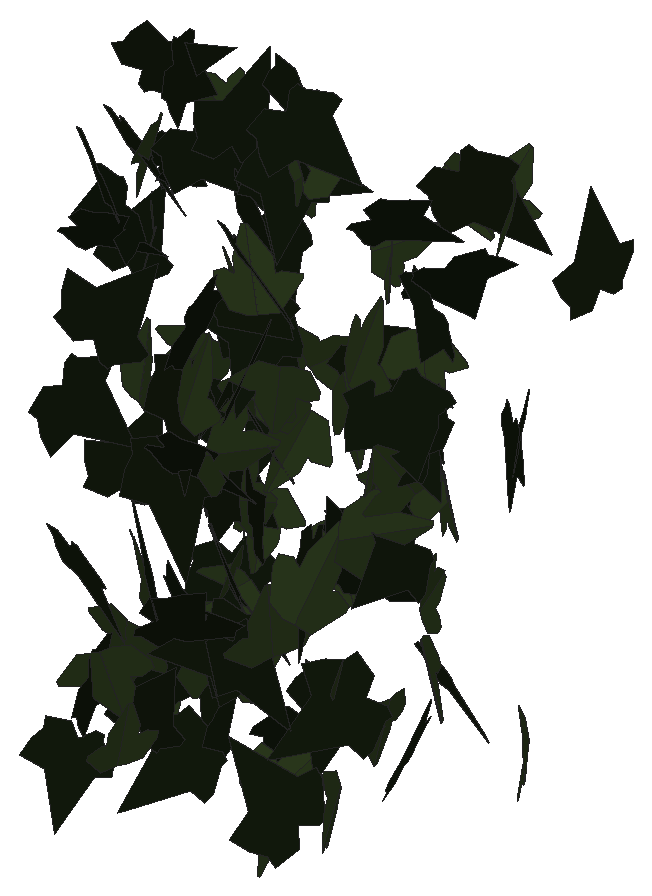
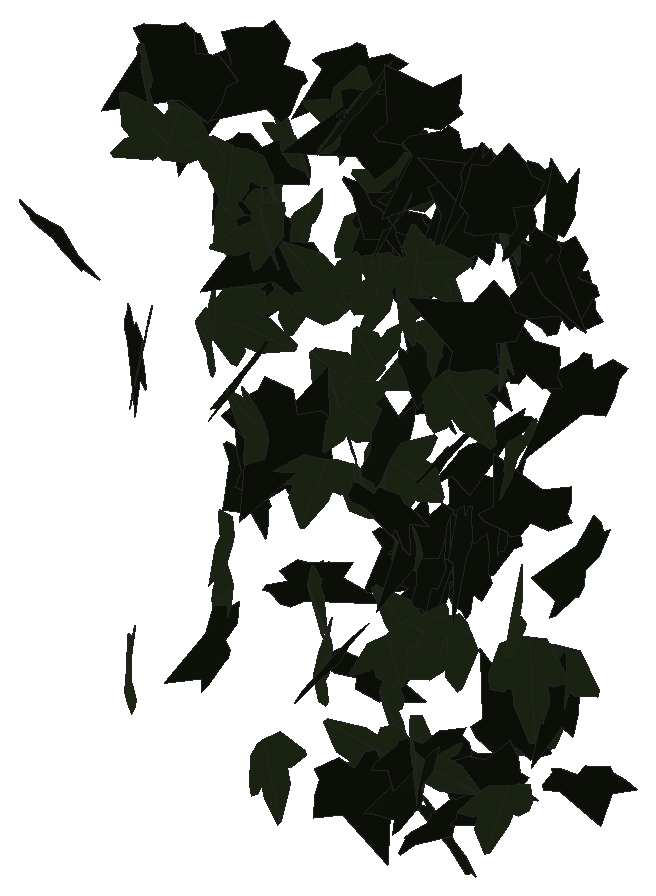
# SketchUp Ruby script. Lengths in inches.
U = 1.inch
M = Sketchup.active_model
def pt(a) = Geom::Point3d.new(a.map { |v| v * U })
def face(e, loops, mat)
  f = e.add_face(loops[0].map { |a| pt(a) })
  loops[1..].each { |l| e.add_face(l.map { |a| pt(a) }).erase! }
  f.material = f.back_material = mat if mat
  f
end
# faces: each face lists its corners as indices into pts; further lists are holes
def faces(e, pts, list, mat = nil) = list.each { |f| face(e, (f[0].is_a?(Array) ? f : [f]).map { |l| l.map { |i| pts[i] } }, mat) }
# xy, xz, yz: faces in a plane at the given z, y or x. An outline is a flat list of corners, or four numbers for a rectangle; further outlines are holes
def ring(l) = l.size == 4 ? [[l[0], l[1]], [l[2], l[1]], [l[2], l[3]], [l[0], l[3]]] : l.each_slice(2).to_a
def flat(e, list, mat, &to3) = list.each { |f| face(e, (f[0].is_a?(Array) ? f : [f]).map { |l| ring(l).map { |u, v| to3.(u, v) } }, mat) }
def xy(e, z, list, mat = nil) = flat(e, list, mat) { |x, y| [x, y, z] }
def xz(e, y, list, mat = nil) = flat(e, list, mat) { |x, z| [x, y, z] }
def yz(e, x, list, mat = nil) = flat(e, list, mat) { |y, z| [x, y, z] }
def lines(e, pts, list) = list.each { |a, b| e.add_line(pt(pts[a]), pt(pts[b])) }
# prism: a flat outline (further loops are holes) pulled along v
def prism(e, loops, v, mat = nil)
  f = face(e, loops, mat); d = Geom::Vector3d.new(v.map { |x| x * U })
  f.pushpull(f.normal.samedirection?(d) ? d.length : -d.length)
end
def box(e, o, s, mat = nil) = prism(e, [[o, [o[0] + s[0], o[1], o[2]], [o[0] + s[0], o[1] + s[1], o[2]], [o[0], o[1] + s[1], o[2]]]], [0, 0, s[2]], mat)
def at(x, y, z, deg = 0) = Geom::Transformation.translation(pt([x, y, z])) * Geom::Transformation.rotation(ORIGIN, Z_AXIS, deg.degrees)
def axes(o, x, y, z) = Geom::Transformation.new([*x, 0, *y, 0, *z, 0, *pt(o).to_a, 1])
def part(name) = M.definitions.add(name)
# library, detail: a bought-in or finely detailed component or shape, given as its bounding box
def library(name, o, s) = part(name).tap { |d| box(d.entities, o, s) }
def detail(e, o, s) = box(e.add_group.entities, o, s)
def put(e, d, t, mat = nil) = e.add_instance(d, t).tap { |i| i.material = mat if mat }
def group(e, t, mat = nil) = e.add_group.tap { |g| g.transformation = t; g.material = mat if mat }.entities
root = M.entities
M.materials.add("efeu1").color = [18, 25, 13]
M.materials.add("efeu2").color = [43, 57, 29]
c1 = part("ivyleaf_9")
p = [[1.54,2.16,1.25],[1.36,2.04,1.19],[-0.21,0.99,0.68],[-0.71,1.11,0.82],[-0.85,0.86,0.67],[-0.8,0.17,0.21],
  [-0.9,-0.01,0.1],[-0.67,-0.16,-0.02],[-0.08,-0.08,-0.05],[-0.03,-0.6,-0.4],[0.65,-0.88,-0.66],[0.83,-0.6,-0.49],
  [1.29,-0.42,-0.43],[1.8125,-0.07,-0.26],[1.21,0.44,0.15]]
faces(c1.entities,p,[[0,1,2,3,4,5,6,7,8,9,10,11,12,13,14]],"efeu1")
c2 = part("ivyleaf_10")
p = [[0,0.5,-0.03],[-0.0625,2.02,-0.43],[-0.19,2.01,-0.46],[-0.54,1.05,-0.29],[-0.52,0.625,-0.18],[-0.83,0.76,-0.28],
  [-1.16,0.64,-0.33],[-1.15,0.33,-0.24],[-0.77,-0.39,0.02],[-0.3,-0.51,0.16],[0.04,-0.48,0.23],[-0.02,2.01,-0.4375],
  [-0.06,2.01,-0.43],[0.04,-0.49,0.23],[0.67,-0.49,0.14],[1.38,0.36,-0.2],[1.375,0.51,-0.24],[0.81,0.65,-0.19],
  [0.62,0.59,-0.15],[0.6,1.09,-0.28],[0.5,1.23,-0.31]]
faces(c2.entities,p,[[0,1,2,3,4,5,6,7,8,9,10],[11,12,0,13,14,15,16,17,18,19,20]],"efeu2")
put(root,c1,axes([566.5,131.97,199.46],[-0.62118,0.17725,0.73217],[0.62302,-0.41261,0.62845],[0.42349,0.867,0.1494]))
put(root,c1,axes([566.02,134.12,201.5],[0.30115,-0.22264,0.87712],[0.9023,0.00334,-0.30895],[0.06905,0.92737,0.21169]))
put(root,c1,axes([566.73,129.25,184.91],[-0.60862,-0.62712,-0.2686],[0.1864,0.19339,-0.8739],[0.65626,-0.63652,-0.00089]))
put(root,c2,axes([567.1,132.19,200.53],[0.16506,-0.4115,-0.84591],[-0.29213,0.79395,-0.44322],[0.89418,0.33534,0.01135]))
put(root,c1,axes([567.51,130.41,202.3125],[0.00641,0.09272,-1.01055],[-0.96381,-0.31575,-0.03509],[-0.31762,0.95998,0.08606]))
put(root,c2,axes([566.76,132.67,185.71],[0.38672,0.88073,0.19755],[0.08149,0.17997,-0.96189],[-0.89893,0.3952,-0.00222]))
put(root,c1,axes([566.47,129.82,201.51],[0.81104,0.26888,0.39363],[0.36374,0.15304,-0.85399],[-0.30811,0.88843,0.02797]))
put(root,c1,axes([566.35,132.93,205.32],[0.18555,-0.02317,0.97755],[0.9739,-0.08478,-0.18686],[0.08762,0.99139,0.00686]))
put(root,c2,axes([567.39,131.24,196.01],[0.00249,0.6236,-0.76732],[-0.15233,0.7584,0.61586],[0.97696,0.11666,0.09798]))
put(root,c1,axes([566.7,130.29,203.21],[0.06086,-0.4186,0.95953],[0.31463,-0.9094,-0.41669],[0.99847,0.31207,0.07282]))
put(root,c2,axes([567.77,135.21,187.71],[0.50512,0.24095,-0.77105],[-0.71518,-0.28945,-0.55897],[-0.37562,0.87514,0.02741]))
put(root,c1,axes([567.61,128.76,187.54],[0.00923,0.05,-1.03786],[-0.76898,0.69835,0.02681],[0.6988,0.76782,0.04321]))
put(root,c2,axes([568,134.8,203.6],[0.41283,0.08387,0.85888],[-0.83837,-0.1867,0.4212],[0.20455,-0.93448,-0.00706]))
put(root,c2,axes([567.66,135.51,188.7],[0.31245,-0.87923,-0.45787],[-0.11998,0.44301,-0.93256],[0.98402,0.33319,0.03168]))
put(root,c1,axes([567.24,132.64,185.49],[-0.14348,-0.21788,0.95466],[0.81574,0.50714,0.23835],[-0.54167,0.82145,0.10606]))
put(root,c1,axes([567.3125,128.03,197.3],[0.22484,-0.41087,-1.00066],[-0.27801,0.96576,-0.45901],[1.04539,0.3452,0.09315]))
put(root,c1,axes([566.89,131.28,204.27],[0.79271,-0.67716,0.24411],[0.18834,-0.15536,-1.04255],[0.69474,0.81477,0.00409]))
put(root,c2,axes([568.02,130.04,188.64],[-1.10864,0.00574,0.38048],[-0.38049,-0.00251,-1.10865],[-0.00462,-1.17211,0.00423]))
put(root,c1,axes([566.92,128.85,191.4],[0.63842,-0.80467,0.3748],[0.26505,-0.2678,-1.02644],[0.84718,0.69017,0.03869]))
put(root,c1,axes([567.46,135.22,185.74],[-0.15802,-0.9049,0.23974],[-0.04819,-0.23495,-0.91856],[0.93488,-0.16506,-0.00683]))
put(root,c1,axes([567.74,132.54,206.02],[0.30579,-0.11355,-0.91049],[-0.66287,0.63625,-0.30197],[0.63443,0.7195,0.12334]))
put(root,c2,axes([567.67,131.57,204.24],[0.37963,-0.89473,0.17404],[0.0831,-0.15377,-0.9718],[0.9077,0.38828,0.01618]))
put(root,c1,axes([567.41,135.54,188.43],[-0.10662,-0.90179,-0.50243],[0.05866,0.49899,-0.90807],[1.03064,-0.12169,-0.00029]))
put(root,c1,axes([567.18,136.02,187.37],[0.71121,-0.65288,0.19575],[0.15137,-0.12455,-0.96538],[0.66457,0.72707,0.0104]))
put(root,c2,axes([567.77,131.06,189.875],[-0.68781,0.62472,0.39731],[0.29297,-0.26837,0.92917],[0.67993,0.74761,0.00155]))
put(root,c1,axes([567.75,130.24,193.375],[-0.60325,-0.14236,0.71503],[0.71227,0.08292,0.61743],[-0.15554,0.93182,0.05429]))
put(root,c2,axes([567.95,129.05,188.04],[-0.81879,-0.68303,-0.25266],[0.19461,0.16114,-1.06628],[0.70178,-0.8416,0.0009]))
put(root,c1,axes([568.61,132.17,193.73],[0.46821,-0.05599,-0.8817],[-0.85711,0.2132,-0.46869],[0.21425,0.97528,0.05184]))
put(root,c2,axes([568.4,134.75,203.56],[0.12329,0.93867,-0.15253],[-0.03341,-0.14943,-0.94664],[-0.9504,0.12702,0.01349]))
put(root,c1,axes([568.65,131.59,203.7],[0.26486,0.77888,0.57502],[0.18712,0.54372,-0.82268],[-0.94989,0.32428,-0.00173]))
put(root,c1,axes([568.15,128.37,199.16],[-0.48726,0.16597,1.02057],[0.90937,-0.46816,0.5103],[0.49209,1.02947,0.06753]))
put(root,c2,axes([568.67,128.875,185.35],[-0.30544,-0.87118,-0.03194],[-0.01062,-0.03012,0.92317],[-0.8717,0.30563,-0.00005]))
put(root,c1,axes([568.85,132.45,183.53],[-0.68715,0.71498,-0.02906],[-0.03079,0.01071,0.99154],[0.71491,0.68768,0.01477]))
put(root,c2,axes([569.39,131.73,197.71],[-0.60682,-0.47004,0.63147],[-0.50445,-0.37991,-0.76754],[0.60434,-0.78908,-0.00661]))
put(root,c1,axes([568.5,130,185.73],[-0.47172,-0.03829,0.85441],[0.72654,-0.53275,0.37725],[0.45124,0.81775,0.28577]))
put(root,c2,axes([569.06,135.04,190.98],[0.34827,0.84637,-0.28373],[-0.10797,-0.26238,-0.91523],[-0.88611,0.36462,0]))
put(root,c1,axes([569.72,131.0625,184.95],[-0.82305,-0.47534,0.30066],[-0.26233,-0.14695,-0.95045],[0.49752,-0.86384,-0.00376]))
put(root,c1,axes([569.76,132.56,195.03],[0.257,-0.90153,-0.3941],[0.11595,-0.37674,0.93742],[-0.97705,-0.28185,0.00758]))
put(root,c2,axes([569.79,133.48,195.71],[-0.01881,-0.66501,0.68277],[0.00919,-0.683,-0.66498],[0.95306,-0.00654,0.01989]))
put(root,c1,axes([570.05,134.36,195.14],[-0.8322,-0.32565,-0.35437],[0.33251,0.12271,-0.89363],[0.34794,-0.89615,0.00641]))
put(root,c1,axes([569.99,132.15,193.4],[0.2135,-0.33568,-0.92615],[-0.49389,0.78348,-0.39782],[0.85236,0.53806,0.00147]))
put(root,c1,axes([570.4,128.19,191.49],[0.17495,-0.63504,0.84748],[-0.13262,0.83907,0.65611],[-1.05067,-0.21166,0.0583]))
put(root,c1,axes([569.64,131.11,205.08],[-0.06299,-0.31077,-1.01968],[0.2765,0.98174,-0.31629],[1.0295,-0.28269,0.02256]))
put(root,c1,axes([569.78,129.8,194.98],[0.07848,-1.1817,-0.18202],[-0.01542,0.1814,-1.1843],[1.19554,0.07991,-0.00333]))
put(root,c1,axes([570.23,129.73,197.87],[-0.7248,-0.13793,-0.87148],[0.84845,0.20057,-0.73739],[0.24215,-1.11561,-0.02483]))
put(root,c2,axes([570.37,130.34,188.53],[-0.21603,-0.26819,-0.96426],[0.55442,0.78922,-0.34372],[0.83327,-0.59464,-0.02129]))
put(root,c1,axes([570.13,129.89,190.1],[-0.00269,-0.16357,0.98202],[0.46756,-0.86719,-0.14316],[0.87893,0.46082,0.07916]))
put(root,c2,axes([571.33,131.3,199.77],[-0.3382,0.54046,-0.77229],[-0.57088,0.53546,0.62473],[0.75008,0.65122,0.12726]))
put(root,c1,axes([570.29,131.59,190.97],[0.14621,-0.34802,0.88683],[0.3282,-0.82389,-0.37743],[0.89435,0.35924,-0.00647]))
put(root,c1,axes([571.125,131.46,198.04],[-0.69858,0.48635,-0.46952],[0.37449,-0.2837,-0.85104],[-0.5628,-0.79245,0.01651]))
put(root,c2,axes([570.31,132.5,192.73],[0.31608,-0.22187,-0.94561],[0.75386,-0.57099,0.38596],[-0.61245,-0.81734,-0.01294]))
put(root,c1,axes([571.3,133.72,185.38],[0.11615,0.74175,-0.59653],[-0.08667,-0.59022,-0.75077],[-0.94791,0.14486,-0.00445]))
put(root,c1,axes([571.08,130.96,205.43],[-0.43405,-0.33463,0.84206],[0.71664,0.44459,0.54608],[-0.5545,0.83654,0.04661]))
put(root,c1,axes([571.16,131.8,192.46],[-0.13819,0.21278,0.98147],[0.25993,-0.94938,0.24243],[0.97005,0.28471,0.07486]))
put(root,c1,axes([570.99,128.2,196.47],[0.99051,0.13202,0.2585],[0.25619,0.03452,-0.99927],[-0.13646,1.02311,0.00036]))
put(root,c1,axes([571.48,130.93,203.73],[0.72763,-0.3147,-0.63293],[-0.55623,0.30558,-0.7914],[0.43616,0.9147,0.04663]))
put(root,c2,axes([571.36,128.7,197.89],[0.97473,-0.54995,-0.13311],[0.12109,-0.05626,1.11913],[-0.55273,-0.98217,0.01043]))
put(root,c1,axes([571,127.68,191.0625],[0.77494,0.33465,0.69773],[0.63568,0.2878,-0.84406],[-0.44128,1.00226,0.0094]))
put(root,c1,axes([571.2,132.4,195.04],[-0.05602,-0.42556,0.89771],[0.42293,-0.8238,-0.36413],[0.89895,0.36106,0.22725]))
put(root,c1,axes([572.0625,130.16,189.6],[-0.0387,-0.71389,-0.7484],[0.03591,-0.7494,0.71298],[-1.03366,0.0007,0.05279]))
put(root,c2,axes([571.29,130.78,188.14],[-0.71966,-0.19837,0.80282],[0.78021,0.18989,0.74632],[-0.27411,1.06131,0.01653]))
put(root,c1,axes([572.11,127.61,201.17],[-0.2349,0.4171,-0.98366],[-0.62481,0.76336,0.47289],[0.8667,0.66336,0.07431]))
put(root,c1,axes([571.93,133.17,206.3],[0.12559,-0.97764,0.57358],[0.18079,-0.55242,-0.98117],[1.11897,0.19898,0.09415]))
put(root,c2,axes([572.39,128.68,196.71],[-0.1548,-0.29786,-1.06539],[0.44851,0.96648,-0.33537],[1.01124,-0.47425,-0.01434]))
put(root,c2,axes([572.73,132.16,196.07],[0.29871,0.71869,-0.68187],[-0.29395,-0.61582,-0.77785],[-0.94608,0.41826,0.02639]))
put(root,c1,axes([572.31,131.75,202.67],[-0.47224,-0.264,-0.81745],[0.8302,0.09933,-0.51169],[0.22064,-0.93881,0.17573]))
put(root,c2,axes([572.71,131.03,197.12],[0.16908,0.77143,-0.57978],[0.15136,0.56013,0.78942],[0.95307,-0.22582,-0.02252]))
put(root,c1,axes([572.17,129.875,202.88],[0.72011,-0.65789,0.31455],[0.22824,-0.21651,-0.97537],[0.69258,0.75539,-0.00562]))
put(root,c2,axes([572.39,131.07,184.39],[0.66465,0.29329,-0.82447],[0.64952,0.52846,0.71161],[0.58642,-0.91774,0.14628]))
put(root,c1,axes([572.42,131.0625,205.1],[0.25264,0.07911,-1.00927],[0.27376,0.99612,0.14661],[0.97464,-0.3003,0.22044]))
put(root,c2,axes([573.16,129.4,201.78],[0.91909,0.4527,0.16181],[-0.14704,-0.06766,1.02453],[0.45771,-0.93077,0.00422]))
put(root,c1,axes([572.53,129.31,190.1],[-0.17577,-0.30886,-0.93652],[0.74225,0.58486,-0.33219],[0.64924,-0.75226,0.12624]))
put(root,c1,axes([572.84,129,198.56],[0.0372,0.90417,0.64244],[-0.06948,-0.63964,0.90425],[1.10699,-0.07053,0.03517]))
put(root,c1,axes([573.25,129.75,201.04],[-0.8651,-0.48561,-0.40044],[0.33289,0.22467,-0.9916],[0.53419,-0.92643,-0.03057]))
put(root,c1,axes([573.1,131.1,205.33],[-0.22663,-0.98888,-0.02007],[0.00515,0.01941,-1.01451],[0.98907,-0.22668,0.00068]))
put(root,c2,axes([573.41,135.07,185.76],[-0.01816,-0.98187,0.02449],[-0.00056,-0.02448,-0.98204],[0.98218,-0.01817,-0.00011]))
put(root,c2,axes([573.37,131.1875,205.03],[0.26939,-0.05167,-1.01039],[0.05465,1.04481,-0.03886],[1.01024,-0.04274,0.27153]))
put(root,c2,axes([573.85,129.02,184.69],[0.29677,-0.31387,-0.91382],[-0.61464,0.67628,-0.43189],[0.74553,0.68249,0.0077]))
put(root,c2,axes([573.45,131.2,204.88],[0.85979,0.56003,0.1115],[-0.1102,-0.03502,1.02564],[0.56029,-0.86628,0.03062]))
put(root,c1,axes([572.86,129.57,201.22],[-0.21072,-0.35699,-0.92094],[0.68272,0.62785,-0.3996],[0.71377,-0.70593,0.11033]))
put(root,c2,axes([573.43,129.63,198.58],[0.22183,0.3763,-1.02635],[0.21841,1.0109,0.41784],[1.07112,-0.28406,0.12736]))
put(root,c1,axes([573.02,131.15,206.9],[0.14887,-0.50956,-0.86644],[0.19229,0.87415,-0.48106],[0.98661,-0.09349,0.22449]))
put(root,c1,axes([573.54,132.37,187.4],[-0.00614,-0.93398,0.44385],[0.03036,-0.44383,-0.93352],[1.03363,0.00749,0.03005]))
put(root,c1,axes([574.875,129.08,185.2],[-0.95646,-0.41932,-0.33083],[-0.30401,-0.1305,1.04434],[-0.43915,1.00361,-0.00243]))
put(root,c2,axes([574.61,128.75,199.87],[-0.84595,-0.55385,0.1592],[-0.12737,-0.09609,-1.01108],[0.56203,-0.85542,0.0105]))
put(root,c2,axes([574.4375,128.67,191.1],[-0.51964,-1.00295,-0.2604],[-0.12226,-0.22993,1.12957],[-1.02896,0.53383,-0.00271]))
put(root,c2,axes([573.78,135.14,196.31],[0.07114,-0.04871,-0.98589],[0.76552,-0.62129,0.08593],[-0.62316,-0.76879,-0.00698]))
put(root,c2,axes([573.98,131.41,198.94],[-0.59061,-0.39241,0.74969],[0.68884,0.30801,0.70389],[-0.49144,0.90331,0.08566]))
put(root,c2,axes([574.26,131.59,193.26],[0.62738,0.76921,0.28156],[0.17761,0.21847,-0.99262],[-0.79963,0.65203,0.00042]))
put(root,c2,axes([574.53,133.6,202.06],[0.16049,-0.11876,-0.96776],[0.4955,0.85462,-0.0227],[0.83972,-0.4816,0.19836]))
put(root,c2,axes([574.4,133.97,202.32],[0.55603,-0.44127,0.74741],[0.61987,-0.41942,-0.70877],[0.60753,0.83179,0.03911]))
put(root,c2,axes([574.74,131.29,188.9375],[0.51957,-0.68468,0.48017],[0.33539,-0.34723,-0.85805],[0.76607,0.6164,0.05]))
put(root,c1,axes([574.61,134.74,197.63],[0.46235,-0.91926,0.05132],[0.02759,-0.04357,-1.02897],[0.92028,0.46315,0.00506]))
put(root,c1,axes([574.9,129.82,193.9375],[-0.5425,-0.02704,-1.02633],[1.00774,-0.23601,-0.52646],[-0.19634,-1.13664,0.13373]))
put(root,c1,axes([575.87,130.88,188.8],[-0.85448,-0.49849,0.46439],[-0.37626,-0.27571,-0.98828],[0.56796,-0.93262,0.04394]))
put(root,c1,axes([575.33,131.5,194.58],[0.76407,0.83812,0.01786],[0.00797,0.0169,-1.13412],[-0.83828,0.76409,0.0055]))
put(root,c1,axes([575.65,131.44,192.35],[0.96129,-0.16489,0.73967],[-0.72278,0.15964,0.97493],[-0.22779,-1.20237,0.028]))
put(root,c2,axes([576.25,133.46,190.97],[-0.02909,0.00098,0.98374],[-0.59962,0.7802,-0.0185],[-0.77988,-0.5999,-0.02246]))
put(root,c2,axes([575.47,130.11,185.6875],[0.0562,-0.18999,1.00594],[0.68039,-0.74582,-0.17887],[0.76491,0.67737,0.0852]))
put(root,c1,axes([575.58,134.45,188.47],[0.8104,-0.56391,0.06856],[0.05601,-0.03954,-0.98729],[0.56529,0.81233,-0.00046]))
put(root,c1,axes([575.73,131.33,200.09],[-0.02039,-0.09909,-1.03263],[0.44866,0.93039,-0.09814],[0.93533,-0.44845,0.02457]))
put(root,c2,axes([576.28,127.63,193.55],[0.35889,0.83852,-0.84906],[0.32898,0.78274,0.91208],[1.14707,-0.48684,0.00406]))
put(root,c2,axes([576.64,129.36,199.82],[-0.11155,1.09921,-0.06423],[0.00299,-0.06426,-1.10485],[-1.10108,-0.11154,0.00351]))
put(root,c2,axes([576.44,133.24,189.41],[-0.45054,0.5092,-0.71379],[0.42383,-0.57605,-0.67845],[-0.76756,-0.61696,0.04435]))
put(root,c2,axes([576.43,134.36,204.54],[0.57163,0.113,0.81816],[0.81126,0.10991,-0.58198],[-0.15499,0.992,-0.02872]))
put(root,c1,axes([576.78,130.41,205.09],[0.77414,0.50657,0.45417],[0.38003,0.24869,-0.92515],[-0.56432,0.86239,0]))
put(root,c2,axes([578.06,131.04,196.6875],[0.24432,0.09094,-1.01984],[-1.02388,0.02318,-0.24322],[0.00145,1.04844,0.09384]))
put(root,c2,axes([577.48,128.76,201.22],[1.01018,-0.55658,-0.25771],[0.22777,-0.12063,1.15335],[-0.56949,-1.03553,0.00415]))
put(root,c2,axes([578.15,128.53,197.96],[0.62401,-0.65114,0.84942],[-0.59337,0.60784,0.90185],[-0.89074,-0.86107,-0.0057]))
put(root,c2,axes([577.8,134.46,204.17],[0.65824,0.49314,-0.58738],[0.46957,0.35288,0.82248],[0.60639,-0.80856,0.00071]))
put(root,c1,axes([579.14,134.0625,197.15],[-0.15094,0.05194,-1.00048],[-0.92207,0.38841,0.15927],[0.39172,0.93429,-0.01059]))
put(root,c2,axes([578.21,127.72,196.42],[-0.10994,-0.10709,-1.14825],[0.73644,0.88112,-0.15269],[0.88747,-0.74444,-0.01554]))
put(root,c1,axes([578.09,132.75,206],[-0.11736,-0.13773,-1.1601],[0.65174,0.95992,-0.1799],[0.96956,-0.66194,-0.01949]))
put(root,c2,axes([578.47,130.33,201.49],[0.97034,0.32831,0.23338],[0.22377,0.06681,-1.02434],[-0.33494,0.99577,-0.00822]))
put(root,c2,axes([578.17,131.74,196.24],[0.12215,-0.22728,1.01631],[0.91334,-0.46827,-0.2145],[0.50036,0.91024,0.14342]))
put(root,c1,axes([578.41,134.62,196.96],[0.14285,-0.06416,-1.00043],[0.90478,-0.42691,0.15657],[-0.43169,-0.91598,-0.0029]))
put(root,c1,axes([578.93,129.32,195.64],[-0.26547,-0.74929,0.72249],[-0.26074,-0.67398,-0.79478],[1.00769,-0.37178,-0.01531]))
put(root,c2,axes([579.375,133.26,205.43],[0.41782,-0.67196,-0.78138],[-0.424,0.6564,-0.79121],[0.93931,0.59519,-0.00958]))
put(root,c2,axes([579.22,128.91,197.87],[-0.43899,-0.74988,-0.66441],[-0.32951,-0.57697,0.86891],[-0.94615,0.54887,0.00566]))
put(root,c1,axes([579.84,128.9,199.24],[-0.39238,0.54894,0.83917],[-0.57396,0.61597,-0.67131],[-0.82226,-0.69192,0.06814]))
put(root,c2,axes([578.6,134.92,186.36],[-0.10356,0.11124,1.08707],[0.8529,-0.67439,0.15026],[0.68312,0.85886,-0.02281]))
put(root,c1,axes([578.86,128.62,200.82],[-0.20799,-0.76517,-0.84013],[0.27516,0.79476,-0.79197],[1.10254,-0.3427,0.03916]))
put(root,c1,axes([579.84,136.83,201.22],[-0.99849,0.26562,-0.29722],[-0.28718,0.07659,1.03321],[0.27644,1.03897,-0.00018]))
put(root,c1,axes([579.375,130.42,204.34],[0.53043,1.01229,-0.1151],[-0.05294,-0.1022,-1.14284],[-1.01743,0.53307,-0.00054]))
put(root,c1,axes([578.98,130.24,203.02],[0.01181,-0.66751,0.82208],[0.16028,-0.81153,-0.66125],[1.04676,0.13179,0.09197]))
put(root,c1,axes([579.87,127.85,189.46],[-0.53616,0.48369,-0.70119],[-0.53538,0.45308,0.72192],[0.66256,0.75753,0.01593]))
